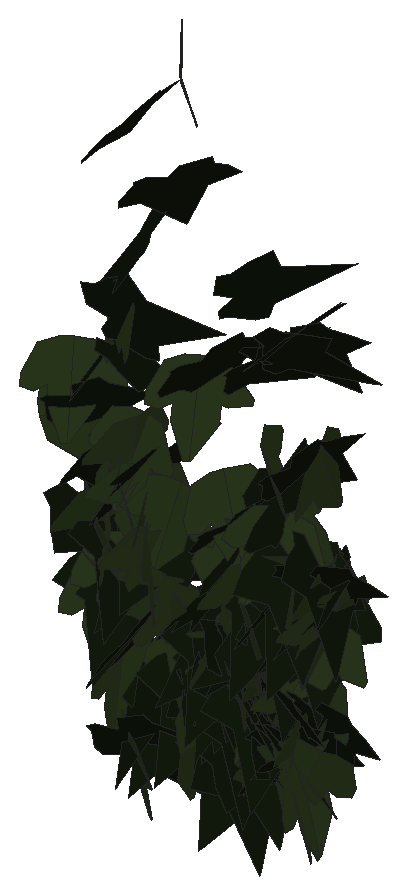
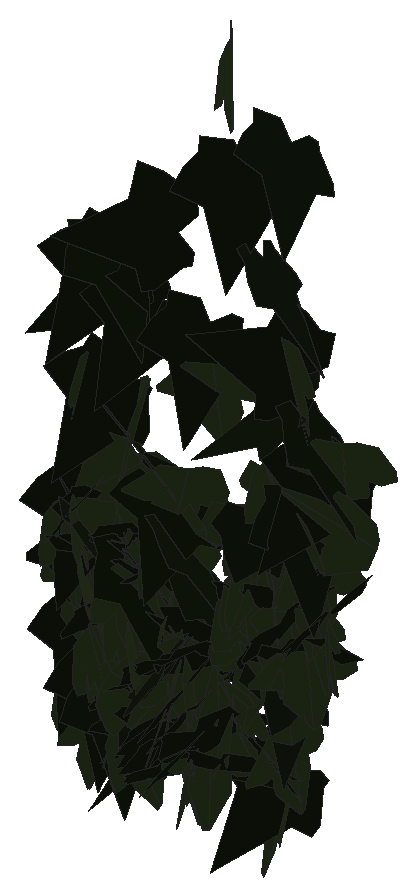
# SketchUp Ruby script. Lengths in inches.
U = 1.inch
M = Sketchup.active_model
def pt(a) = Geom::Point3d.new(a.map { |v| v * U })
def face(e, loops, mat)
  f = e.add_face(loops[0].map { |a| pt(a) })
  loops[1..].each { |l| e.add_face(l.map { |a| pt(a) }).erase! }
  f.material = f.back_material = mat if mat
  f
end
# faces: each face lists its corners as indices into pts; further lists are holes
def faces(e, pts, list, mat = nil) = list.each { |f| face(e, (f[0].is_a?(Array) ? f : [f]).map { |l| l.map { |i| pts[i] } }, mat) }
# xy, xz, yz: faces in a plane at the given z, y or x. An outline is a flat list of corners, or four numbers for a rectangle; further outlines are holes
def ring(l) = l.size == 4 ? [[l[0], l[1]], [l[2], l[1]], [l[2], l[3]], [l[0], l[3]]] : l.each_slice(2).to_a
def flat(e, list, mat, &to3) = list.each { |f| face(e, (f[0].is_a?(Array) ? f : [f]).map { |l| ring(l).map { |u, v| to3.(u, v) } }, mat) }
def xy(e, z, list, mat = nil) = flat(e, list, mat) { |x, y| [x, y, z] }
def xz(e, y, list, mat = nil) = flat(e, list, mat) { |x, z| [x, y, z] }
def yz(e, x, list, mat = nil) = flat(e, list, mat) { |y, z| [x, y, z] }
def lines(e, pts, list) = list.each { |a, b| e.add_line(pt(pts[a]), pt(pts[b])) }
# prism: a flat outline (further loops are holes) pulled along v
def prism(e, loops, v, mat = nil)
  f = face(e, loops, mat); d = Geom::Vector3d.new(v.map { |x| x * U })
  f.pushpull(f.normal.samedirection?(d) ? d.length : -d.length)
end
def box(e, o, s, mat = nil) = prism(e, [[o, [o[0] + s[0], o[1], o[2]], [o[0] + s[0], o[1] + s[1], o[2]], [o[0], o[1] + s[1], o[2]]]], [0, 0, s[2]], mat)
def at(x, y, z, deg = 0) = Geom::Transformation.translation(pt([x, y, z])) * Geom::Transformation.rotation(ORIGIN, Z_AXIS, deg.degrees)
def axes(o, x, y, z) = Geom::Transformation.new([*x, 0, *y, 0, *z, 0, *pt(o).to_a, 1])
def part(name) = M.definitions.add(name)
# library, detail: a bought-in or finely detailed component or shape, given as its bounding box
def library(name, o, s) = part(name).tap { |d| box(d.entities, o, s) }
def detail(e, o, s) = box(e.add_group.entities, o, s)
def put(e, d, t, mat = nil) = e.add_instance(d, t).tap { |i| i.material = mat if mat }
def group(e, t, mat = nil) = e.add_group.tap { |g| g.transformation = t; g.material = mat if mat }.entities
root = M.entities
M.materials.add("efeu1").color = [18, 25, 13]
M.materials.add("efeu2").color = [43, 57, 29]
c1 = part("ivyleaf_10")
p = [[0,0.5,-0.03],[-0.0625,2.02,-0.43],[-0.19,2.01,-0.46],[-0.54,1.05,-0.29],[-0.52,0.625,-0.18],[-0.83,0.76,-0.28],
  [-1.16,0.64,-0.33],[-1.15,0.33,-0.24],[-0.77,-0.39,0.02],[-0.3,-0.51,0.16],[0.04,-0.48,0.23],[-0.02,2.01,-0.4375],
  [-0.06,2.01,-0.43],[0.04,-0.49,0.23],[0.67,-0.49,0.14],[1.38,0.36,-0.2],[1.375,0.51,-0.24],[0.81,0.65,-0.19],
  [0.62,0.59,-0.15],[0.6,1.09,-0.28],[0.5,1.23,-0.31]]
faces(c1.entities,p,[[0,1,2,3,4,5,6,7,8,9,10],[11,12,0,13,14,15,16,17,18,19,20]],"efeu2")
c2 = part("ivyleaf_9")
p = [[1.54,2.16,1.25],[1.36,2.04,1.19],[-0.21,0.99,0.68],[-0.71,1.11,0.82],[-0.85,0.86,0.67],[-0.8,0.17,0.21],
  [-0.9,-0.01,0.1],[-0.67,-0.16,-0.02],[-0.08,-0.08,-0.05],[-0.03,-0.6,-0.4],[0.65,-0.88,-0.66],[0.83,-0.6,-0.49],
  [1.29,-0.42,-0.43],[1.8125,-0.07,-0.26],[1.21,0.44,0.15]]
faces(c2.entities,p,[[0,1,2,3,4,5,6,7,8,9,10,11,12,13,14]],"efeu1")
put(root,c1,axes([30.3,224.12,225.6],[0.37736,-0.315,-0.09151],[-0.05841,0.07272,-0.49122],[0.32278,0.38142,0.01809]))
put(root,c2,axes([31.09,224.05,229.85],[-0.32098,0.38105,-0.04203],[0.0204,-0.03777,-0.49815],[-0.38282,-0.32151,0.0087]))
put(root,c1,axes([32.95,224.22,225.7],[0.4115,-0.27207,0.08154],[0.06408,-0.05092,-0.49326],[0.27671,0.41639,-0.00704]))
put(root,c1,axes([29.88,224.12,227.76],[0.44345,0.23059,0.01335],[0.00957,0.01054,-0.4998],[-0.23078,0.44353,0.00493]))
put(root,c1,axes([30.82,224.17,227.08],[0.49787,-0.03559,-0.02934],[-0.02948,-0.0009,-0.49913],[0.03547,0.49873,-0.003]))
put(root,c1,axes([31.14,224.18,225.69],[-0.17474,-0.46526,0.05474],[-0.02065,-0.05071,-0.49699],[0.46802,-0.17595,-0.00149]))
put(root,c1,axes([30.83,224.13,227.14],[-0.12225,-0.48376,-0.0321],[0.01251,0.02994,-0.49895],[0.48466,-0.1228,0.00478]))
put(root,c2,axes([30.59,224.0625,228.59],[0.23955,-0.05802,0.43503],[0.42307,-0.10129,-0.24648],[0.11673,0.48618,0.00056]))
put(root,c1,axes([32.96,224.18,226.5],[0.42461,0.19838,-0.17422],[-0.16939,-0.04839,-0.46794],[-0.20252,0.4564,0.02611]))
put(root,c1,axes([32.49,224.13,225.16],[-0.31015,0.36238,-0.14995],[0.0853,-0.12427,-0.47674],[-0.38279,-0.32131,0.01526]))
put(root,c1,axes([33.67,224.24,225.55],[-0.07005,-0.48173,0.11414],[-0.03359,-0.11038,-0.48651],[0.49393,-0.07583,-0.0169]))
put(root,c2,axes([30.58,224.36,225.09],[-0.32012,-0.37428,-0.08623],[0.09357,0.03287,-0.49007],[0.37251,-0.3299,0.049]))
put(root,c1,axes([31.75,224.14,228.16],[0.42086,0.26939,-0.01753],[-0.01578,-0.00786,-0.49969],[-0.2695,0.42115,0.00189]))
put(root,c1,axes([30.37,224.11,226.1],[-0.14844,-0.47359,-0.06063],[0.00619,0.06157,-0.49616],[0.47742,-0.14805,-0.01241]))
put(root,c2,axes([31.54,223.89,230.85],[0.18063,0.46243,-0.0594],[-0.05589,-0.04177,-0.49511],[-0.46287,0.1855,0.0366]))
put(root,c1,axes([31.22,224.16,225.15],[-0.41234,-0.21138,0.18786],[-0.16948,-0.08117,-0.46334],[0.22638,-0.44579,-0.00471]))
put(root,c2,axes([32.92,224.22,225.35],[-0.4789,0.12972,-0.06187],[0.06277,-0.00483,-0.49602],[-0.12929,-0.48285,-0.01166]))
put(root,c2,axes([30.84,223.9,223.19],[0.45207,0.21327,0.01211],[0.01117,0.0047,-0.49985],[-0.21332,0.45221,-0.00052]))
put(root,c2,axes([32.83,224.35,225.65],[-0.39468,-0.2935,-0.08994],[0.0732,0.0523,-0.49184],[0.29812,-0.4014,0.00169]))
put(root,c2,axes([33.04,223.97,224.45],[0.43303,0.03926,-0.24687],[-0.24766,0.00037,-0.43436],[-0.03393,0.49846,0.01977]))
put(root,c1,axes([31.9,223.77,223.41],[0.07883,-0.08771,-0.48589],[0.02445,0.49214,-0.08487],[0.49314,-0.01038,0.08188]))
put(root,c2,axes([30.91,223.84,224.4375],[-0.04253,0.47968,0.13452],[-0.0004,0.13497,-0.48144],[-0.49819,-0.04106,-0.01109]))
put(root,c1,axes([31.78,223.89,232.26],[-0.17235,0.1208,0.45354],[-0.37587,0.25384,-0.21045],[-0.2811,-0.41349,0.00331]))
put(root,c1,axes([31.39,224.13,226.38],[0.48688,0.0507,-0.10186],[-0.10875,0.07571,-0.48212],[-0.03347,0.49163,0.08475]))
put(root,c2,axes([32.35,224.3,223.28],[0.02509,-0.48999,-0.09631],[-0.01226,0.0958,-0.49058],[0.49922,0.02698,-0.00721]))
put(root,c2,axes([32.07,223.88,228.59],[0.1374,0.48057,0.01328],[-0.00137,0.0142,-0.4998],[-0.48075,0.1373,0.00522]))
put(root,c1,axes([33.49,224.2,223.57],[-0.39481,-0.23216,0.20056],[-0.17451,-0.09888,-0.458],[0.25233,-0.43165,-0.00295]))
put(root,c1,axes([30.6,224.17,225.37],[0.39451,0.3071,-0.00734],[-0.00136,-0.01019,-0.49989],[-0.30719,0.39444,-0.0072]))
put(root,c2,axes([33.23,224.29,226.15],[-0.22625,-0.39492,-0.207],[0.10151,0.1804,-0.45514],[0.43417,-0.24798,-0.00145]))
put(root,c1,axes([30.9375,224.23,226.46],[-0.28678,-0.4043,0.06557],[0.01237,-0.08856,-0.49194],[0.4094,-0.28053,0.06079]))
put(root,c1,axes([30.66,224.125,228.77],[0.3659,-0.3019,-0.15803],[-0.08981,0.13823,-0.47204],[0.32871,0.37383,0.04693]))
put(root,c2,axes([30.52,224.47,225.52],[-0.08283,-0.48019,0.11204],[-0.02176,-0.10994,-0.48728],[0.49261,-0.0856,-0.00268]))
put(root,c2,axes([30.875,223.87,231.37],[0.00294,0.48423,0.12456],[-0.04367,0.12434,-0.48232],[-0.49808,-0.00804,0.04302]))
put(root,c1,axes([30.82,224.09,222.96],[-0.35903,0.34793,0.00695],[-0.00562,0.0042,-0.49995],[-0.34795,-0.35907,0.00089]))
put(root,c2,axes([32.99,224.38,225.24],[-0.48549,-0.07263,0.09499],[-0.08683,-0.05897,-0.48886],[0.08221,-0.49117,0.04465]))
put(root,c1,axes([32.42,224.23,225.71],[-0.0456,-0.4977,0.01456],[0.01355,-0.01586,-0.49956],[0.49773,-0.04517,0.01494]))
put(root,c1,axes([32.125,224.22,223.23],[0.44772,-0.22255,-0.00387],[0.01422,0.03727,-0.49841],[0.22213,0.44619,0.0397]))
put(root,c1,axes([32.17,224.34,224.6],[-0.21002,0.28183,-0.35562],[0.18143,-0.30702,-0.35046],[-0.41591,-0.27624,0.02669]))
put(root,c1,axes([33.61,224.23,225.28],[0.42428,0.15566,-0.21389],[-0.21991,-0.01717,-0.44871],[-0.14704,0.47484,0.0539]))
put(root,c1,axes([31.91,224.34,224.39],[0.15364,-0.44944,0.15621],[0.1286,-0.11881,-0.46834],[0.4581,0.18409,0.07909]))
put(root,c1,axes([30.36,224.2,224.93],[0.31245,0.38741,-0.04784],[-0.02493,-0.04134,-0.49766],[-0.38956,0.31337,-0.00651]))
put(root,c1,axes([30.64,224.11,226.43],[-0.29534,0.40332,-0.01027],[0.00966,-0.00566,-0.49987],[-0.40334,-0.29546,-0.00445]))
put(root,c2,axes([32.1,224.36,224.58],[0.24039,-0.43027,0.08413],[0.05534,-0.0654,-0.49261],[0.43491,0.24615,0.01618]))
put(root,c1,axes([31.04,224.22,225.75],[-0.14125,-0.47955,-0.00897],[-0.01111,0.01262,-0.49972],[0.4795,-0.14097,-0.01422]))
put(root,c2,axes([33.24,224.48,225.71],[-0.3202,-0.38331,-0.02322],[0.07261,-0.03074,-0.49374],[0.37709,-0.31957,0.07535]))
put(root,c1,axes([31.07,224.22,225.71],[-0.12149,0.47249,-0.1095],[-0.02453,-0.11873,-0.48508],[-0.4844,-0.11249,0.05203]))
put(root,c1,axes([30.4,224.28,226.76],[0.38348,-0.3207,0.00968],[0.00724,-0.00643,-0.49991],[0.32076,0.38355,-0.00029]))
put(root,c2,axes([33.62,224.38,225.95],[-0.42545,0.1523,-0.21401],[0.15111,-0.19129,-0.43655],[-0.21484,-0.43614,0.11674]))
put(root,c2,axes([32.61,224.49,224.01],[-0.16533,-0.4717,0.01291],[0.07463,-0.03965,-0.49281],[0.46594,-0.16102,0.08352]))
put(root,c2,axes([32.59,223.88,229.66],[0.24858,0.08526,0.42537],[0.34881,0.25222,-0.2544],[-0.25795,0.42322,0.06591]))
put(root,c2,axes([33.62,224.06,224.33],[0.42185,0.14319,-0.22703],[-0.21152,-0.08302,-0.44538],[-0.16525,0.47181,-0.00947]))
put(root,c2,axes([32.2,224.57,223.12],[-0.24171,-0.42033,0.12206],[0.03998,-0.16005,-0.472],[0.43587,-0.21841,0.11098]))
put(root,c2,axes([33.45,224.46,226.09],[0.09075,-0.48262,0.09406],[0.01713,-0.09248,-0.49107],[0.4914,0.09235,-0.00025]))
put(root,c1,axes([30.34,224.07,225.65],[-0.33206,0.1992,0.31632],[-0.30377,0.10278,-0.38361],[-0.21785,-0.44694,0.05276]))
put(root,c2,axes([32.21,224.41,224.91],[-0.49278,-0.08259,0.01859],[-0.01949,0.00386,-0.4996],[0.08238,-0.49312,-0.00702]))
put(root,c1,axes([33.18,224.16,223.21],[-0.28386,0.41122,-0.01798],[0.00756,-0.01663,-0.49967],[-0.41154,-0.28395,0.00323]))
put(root,c2,axes([33.18,224,226.92],[-0.17919,0.31908,0.34071],[-0.23184,0.25591,-0.3616],[-0.40514,-0.28757,0.05624]))
put(root,c1,axes([31.07,224.3125,225.48],[-0.30041,-0.38414,0.11041],[-0.05357,-0.09818,-0.48733],[0.39608,-0.30463,0.01783]))
put(root,c2,axes([32.08,224.24,225.54],[-0.3547,0.34353,-0.07856],[0.02384,-0.08781,-0.49165],[-0.35159,-0.35252,0.04591]))
put(root,c2,axes([31.02,224.47,225.72],[-0.46291,-0.1783,-0.06266],[0.07362,-0.01743,-0.49424],[0.17406,-0.46681,0.04238]))
put(root,c2,axes([29.95,224.29,225.8],[0.20104,-0.43729,-0.13549],[0.00157,0.14864,-0.47739],[0.4578,0.19153,0.06114]))
put(root,c2,axes([32.03,224.57,224.56],[-0.29481,-0.40152,0.04325],[0.03003,-0.0752,-0.4934],[0.40272,-0.28832,0.06845]))
put(root,c2,axes([30.1,223.97,227.38],[0.39835,0.29564,0.0626],[0.04616,0.04283,-0.49602],[-0.29864,0.40096,0.00683]))
put(root,c2,axes([33.32,224.0625,229.33],[-0.07894,0.49366,-0.00841],[-0.08923,-0.02264,-0.49145],[-0.4856,-0.07609,0.09167]))
put(root,c2,axes([30.62,224.13,228.15],[0.43667,-0.24113,-0.03424],[0.05829,0.17173,-0.46595],[0.23647,0.40295,0.17809]))
put(root,c1,axes([31.34,224.32,224.19],[0.45556,-0.20579,-0.01053],[-0.00913,0.00538,-0.49989],[0.20586,0.45565,0.00115]))
put(root,c2,axes([30.98,224.45,223.8],[-0.41922,-0.04152,-0.26932],[0.27243,-0.05284,-0.41592],[0.00607,-0.49546,0.06693]))
put(root,c1,axes([30.85,224.29,226.16],[0.28119,-0.41201,-0.03427],[0.02833,0.06055,-0.49551],[0.41246,0.27673,0.0574]))
put(root,c2,axes([33.22,224.08,223.86],[0.33242,0.31746,-0.19676],[-0.16327,-0.11339,-0.45879],[-0.33592,0.36927,0.02827]))
put(root,c2,axes([32.98,224,229.04],[0.44205,0.12969,0.19434],[0.17138,0.10267,-0.45835],[-0.1588,0.47185,0.04632]))
put(root,c2,axes([32.28,224.53,223.71],[-0.02222,-0.49686,0.05137],[-0.00734,-0.05109,-0.49733],[0.49945,-0.02286,-0.00502]))
put(root,c2,axes([31.02,224.37,226.75],[-0.21855,0.3427,-0.29119],[0.03195,-0.31111,-0.39012],[-0.44857,-0.18912,0.11408]))
put(root,c2,axes([30.37,224.2,228.0625],[-0.27823,0.41341,-0.04095],[0.02378,-0.03336,-0.49832],[-0.41476,-0.27924,-0.0011]))
put(root,c1,axes([32.89,224.11,227.46],[-0.28794,0.37203,0.16935],[-0.09945,0.13717,-0.47042],[-0.39648,-0.30459,-0.00499]))
put(root,c1,axes([31.89,224.48,223.1875],[-0.18009,0.32384,-0.3357],[0.08134,-0.33254,-0.36442],[-0.45929,-0.18587,0.06709]))
put(root,c2,axes([32.66,224.3,223.875],[0.41182,-0.28354,-0.00234],[0.00024,0.00447,-0.49998],[0.28355,0.41181,0.00381]))
put(root,c2,axes([32.23,224.56,224.36],[-0.3465,-0.36039,-0.00764],[0.00651,0.00434,-0.49994],[0.36041,-0.34656,0.00168]))
put(root,c2,axes([30.46,224.1,226.83],[-0.0126,0.49848,-0.0368],[-0.00493,-0.03693,-0.49861],[-0.49982,-0.01221,0.00585]))
put(root,c1,axes([32.12,224.25,226.71],[0.31555,0.37791,0.08725],[0.05988,0.06366,-0.4923],[-0.3832,0.32115,-0.00509]))
put(root,c1,axes([33.34,224.2,223.27],[0.00586,0.49572,0.06499],[-0.04238,0.06525,-0.49391],[-0.49817,0.00028,0.04279]))
put(root,c1,axes([32.74,224.48,223.27],[0.00162,-0.47318,0.16155],[-0.00062,-0.16155,-0.47318],[0.5,0.00134,-0.00111]))
put(root,c1,axes([33.29,224.3125,224.04],[0.09689,-0.48499,-0.0735],[-0.01084,0.07278,-0.49456],[0.4904,0.09743,0.00359]))
put(root,c1,axes([33.12,224.26,226],[-0.42621,-0.25689,-0.0485],[0.03613,0.03399,-0.49753],[0.25892,-0.42761,-0.0104]))
put(root,c1,axes([30.53,224.3125,223.89],[0.05572,0.49032,-0.08049],[-0.10755,-0.06717,-0.48365],[-0.48511,0.07121,0.09798]))
put(root,c1,axes([33.48,224.37,224.42],[0.47117,-0.15699,-0.0579],[-0.055,0.01809,-0.49664],[0.15803,0.47437,-0.00022]))
put(root,c1,axes([29.59,224.29,226.875],[0.162,-0.02458,-0.47239],[0.4711,-0.03664,0.16346],[-0.04265,-0.49805,0.01129]))
put(root,c1,axes([32.67,224.64,224.06],[-0.17531,-0.28929,0.36821],[0.03497,-0.40016,-0.29774],[0.46695,-0.07865,0.16054]))
put(root,c2,axes([32.44,224.43,223.59],[-0.14923,-0.40372,-0.25445],[0.15252,0.21227,-0.42624],[0.45218,-0.20483,0.0598]))
put(root,c1,axes([32.25,224.36,224.15],[-0.32216,0.35961,-0.12996],[0.03065,-0.1451,-0.4775],[-0.38114,-0.31563,0.07144]))
put(root,c1,axes([32.15,224.41,224.45],[-0.3724,-0.22472,0.24661],[-0.20736,-0.13363,-0.43491],[0.26138,-0.42619,0.00633]))
put(root,c1,axes([32.12,224.18,225.96],[0.27026,0.08883,0.41118],[0.32741,0.26244,-0.2719],[-0.26413,0.41621,0.08369]))
put(root,c2,axes([31.82,224.42,223.95],[0.18928,-0.44951,-0.11006],[-0.01285,0.11376,-0.48672],[0.46261,0.18708,0.03151]))
put(root,c2,axes([33.25,224.08,229.2],[0.3952,0.30612,0.01056],[0.00178,0.01495,-0.49977],[-0.3063,0.39505,0.01073]))
put(root,c1,axes([31.9,224.25,224.19],[-0.44856,0.21757,0.0382],[-0.03287,0.01976,-0.49853],[-0.21843,-0.44975,-0.00343]))
put(root,c1,axes([33.7,224.39,225.72],[-0.07162,-0.49459,-0.01591],[0.00932,0.01472,-0.4997],[0.49476,-0.07188,0.00711]))
put(root,c2,axes([33.49,224.13,226.1],[0.36843,0.31241,-0.12907],[-0.12603,-0.0502,-0.48124],[-0.31365,0.38714,0.04175]))
put(root,c1,axes([32.61,224.33,224.62],[0.48731,0.10401,0.04139],[0.02096,0.09684,-0.49009],[-0.10996,0.47938,0.09002]))
put(root,c1,axes([33.45,224.43,225.9375],[0.12988,-0.48279,0.00659],[0.00665,-0.00504,-0.49993],[0.48279,0.12995,0.00511]))
put(root,c2,axes([31.92,224.58,224.17],[0.12817,-0.48095,0.04753],[-0.00134,-0.04953,-0.49754],[0.48329,0.12741,-0.01399]))
put(root,c2,axes([33.13,224.15,223.54],[0.02411,0.49807,-0.03663],[-0.02129,-0.03561,-0.49828],[-0.49896,0.02558,0.01949]))
put(root,c1,axes([33.12,224.48,224.34],[-0.11552,-0.47625,0.09921],[-0.02261,-0.0966,-0.49006],[0.48595,-0.1177,0.00078]))
put(root,c1,axes([32.64,224.4375,224.57],[0.155,-0.47537,-0.00127],[0.00396,0.00262,-0.49998],[0.47535,0.15499,0.00458]))
put(root,c1,axes([32.04,224.24,224.33],[-0.29851,-0.24056,-0.32097],[0.28717,0.15116,-0.38037],[0.28004,-0.41144,0.04792]))
put(root,c2,axes([32.9375,224.64,225.05],[-0.10555,-0.48834,0.01956],[-0.00425,-0.01909,-0.49962],[0.48871,-0.10563,-0.00012]))
put(root,c1,axes([32.87,224.43,224.81],[0.03612,-0.49867,-0.00445],[-0.00225,0.0043,-0.49998],[0.49869,0.03614,-0.00193]))
put(root,c1,axes([31.0625,224.3,224.91],[-0.48275,0.12283,0.04315],[-0.04166,0.01127,-0.49813],[-0.12334,-0.48455,-0.00064]))
put(root,c1,axes([33.53,224.23,227.6],[0.06837,-0.42102,-0.26089],[0.03995,0.2672,-0.42073],[0.49369,0.03669,0.07018]))
put(root,c2,axes([31.22,224.66,223.56],[-0.41582,-0.26712,-0.07577],[0.12146,-0.05231,-0.48219],[0.24968,-0.41942,0.10839]))
put(root,c2,axes([31.57,224.68,223.82],[-0.29618,-0.40003,0.04749],[-0.03474,-0.03336,-0.49768],[0.40134,-0.2981,-0.00803]))
put(root,c1,axes([32.85,224.33,226.67],[0.29455,0.09936,0.39162],[0.36454,0.1436,-0.31062],[-0.1742,0.46852,0.01216]))
put(root,c1,axes([33.45,224.41,224.46],[0.33843,-0.34549,-0.12688],[-0.08652,0.09285,-0.48362],[0.35774,0.34931,0.00307]))
put(root,c1,axes([31.47,224.38,223.97],[-0.38793,0.30953,-0.06084],[0.01738,-0.07532,-0.49399],[-0.31498,-0.38538,0.04768]))
put(root,c2,axes([32.19,224.33,226.02],[-0.33497,0.36902,0.04026],[-0.05659,0.00284,-0.49678],[-0.36687,-0.33736,0.03986]))
put(root,c2,axes([32.34,224.28,223.4375],[0.20649,-0.31421,-0.3296],[-0.05563,0.34178,-0.36068],[0.45196,0.18562,0.10619]))
put(root,c2,axes([33.28,224.05,227.52],[0.22262,0.41439,0.16947],[0.06716,0.15621,-0.4702],[-0.44264,0.23212,0.01389]))
put(root,c1,axes([33.3125,224.53,225.31],[0.201,-0.4547,0.05333],[0.01524,-0.05157,-0.4971],[0.45757,0.20146,-0.00687]))
put(root,c2,axes([32.67,224.47,223.59],[0.26832,-0.41056,-0.09718],[-0.06186,0.07564,-0.49036],[0.41734,0.27517,-0.0102]))
put(root,c2,axes([33.39,224.58,225.52],[-0.31335,-0.32053,-0.22152],[0.1656,0.14775,-0.44805],[0.35268,-0.35416,0.01356]))
put(root,c2,axes([31.78,224.67,223.49],[0.077,-0.48755,0.07977],[0.03642,-0.07491,-0.49301],[0.49269,0.08174,0.02398]))
put(root,c1,axes([32.18,224.58,223.91],[-0.16904,0.34437,-0.32067],[0.1362,-0.29035,-0.3836],[-0.45042,-0.21704,0.00436]))
put(root,c2,axes([32.3,224.1,226.41],[0.16111,0.46055,0.10926],[-0.02799,0.12449,-0.48345],[-0.4725,0.14966,0.06589]))
put(root,c1,axes([32.66,224.49,225.32],[-0.28092,-0.41173,0.03951],[0.02519,-0.0647,-0.49516],[0.41285,-0.27621,0.05709]))
put(root,c2,axes([32.86,224.3,225.49],[-0.15985,0.46944,-0.06383],[0.02784,-0.05794,-0.49585],[-0.47294,-0.16208,-0.00761]))
put(root,c1,axes([31.66,224.4,223.52],[-0.49012,-0.06251,0.07666],[-0.0743,-0.02319,-0.4939],[0.0653,-0.49553,0.01344]))
put(root,c2,axes([32.17,224.57,224.47],[0.2687,-0.41611,0.06819],[0.05471,-0.04577,-0.49489],[0.4181,0.27341,0.02094]))
put(root,c2,axes([32.72,224.09,228.75],[0.20635,0.43272,0.14202],[0.05399,0.13158,-0.47935],[-0.45222,0.21316,0.00758]))
